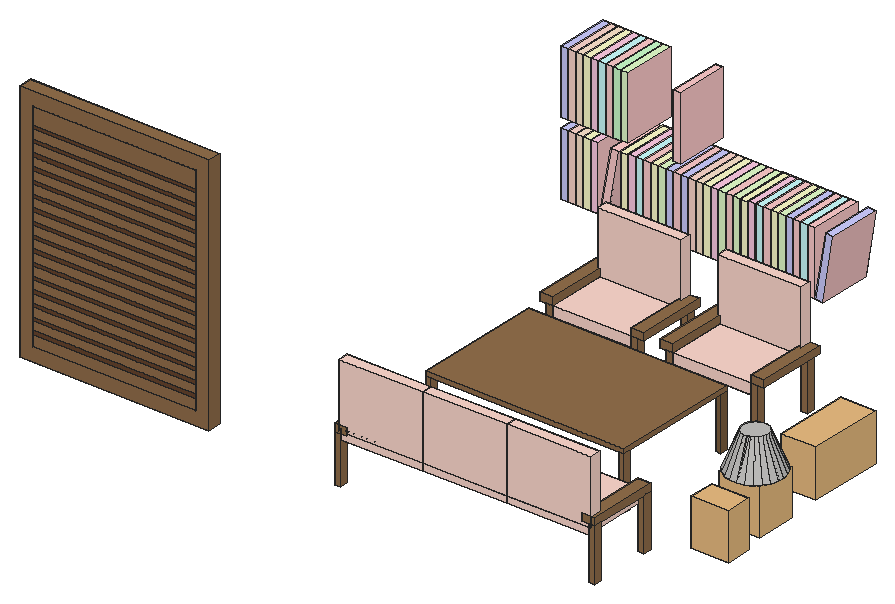
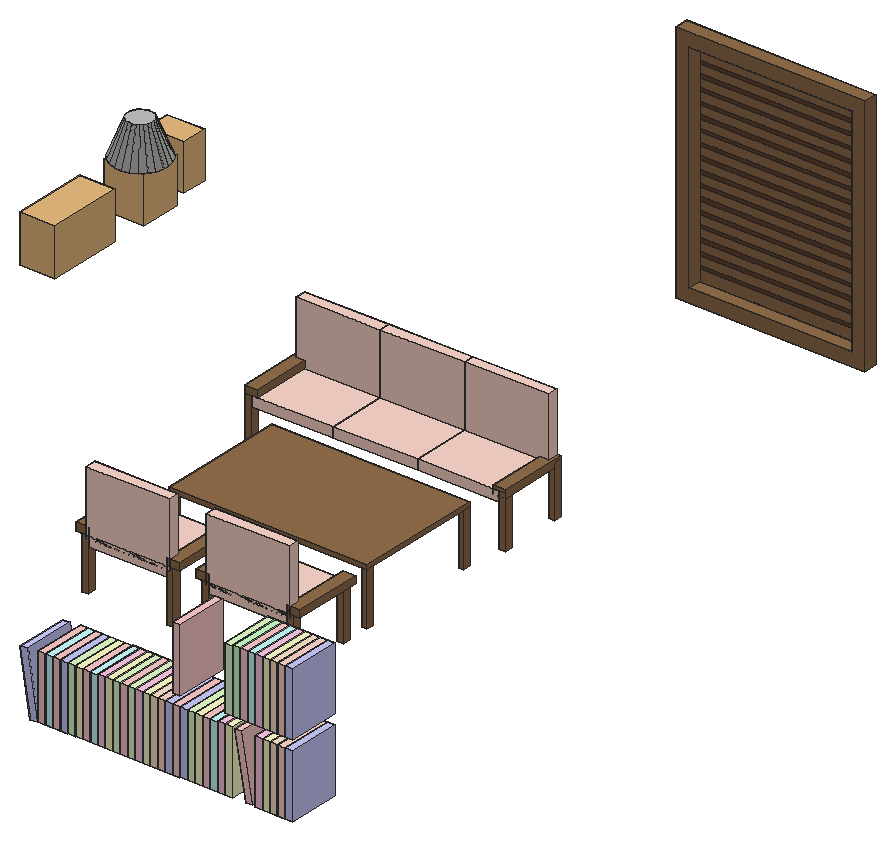
# SketchUp Ruby script. Lengths in inches.
U = 1.inch
M = Sketchup.active_model
def pt(a) = Geom::Point3d.new(a.map { |v| v * U })
def face(e, loops, mat)
  f = e.add_face(loops[0].map { |a| pt(a) })
  loops[1..].each { |l| e.add_face(l.map { |a| pt(a) }).erase! }
  f.material = f.back_material = mat if mat
  f
end
# faces: each face lists its corners as indices into pts; further lists are holes
def faces(e, pts, list, mat = nil) = list.each { |f| face(e, (f[0].is_a?(Array) ? f : [f]).map { |l| l.map { |i| pts[i] } }, mat) }
# xy, xz, yz: faces in a plane at the given z, y or x. An outline is a flat list of corners, or four numbers for a rectangle; further outlines are holes
def ring(l) = l.size == 4 ? [[l[0], l[1]], [l[2], l[1]], [l[2], l[3]], [l[0], l[3]]] : l.each_slice(2).to_a
def flat(e, list, mat, &to3) = list.each { |f| face(e, (f[0].is_a?(Array) ? f : [f]).map { |l| ring(l).map { |u, v| to3.(u, v) } }, mat) }
def xy(e, z, list, mat = nil) = flat(e, list, mat) { |x, y| [x, y, z] }
def xz(e, y, list, mat = nil) = flat(e, list, mat) { |x, z| [x, y, z] }
def yz(e, x, list, mat = nil) = flat(e, list, mat) { |y, z| [x, y, z] }
def lines(e, pts, list) = list.each { |a, b| e.add_line(pt(pts[a]), pt(pts[b])) }
# prism: a flat outline (further loops are holes) pulled along v
def prism(e, loops, v, mat = nil)
  f = face(e, loops, mat); d = Geom::Vector3d.new(v.map { |x| x * U })
  f.pushpull(f.normal.samedirection?(d) ? d.length : -d.length)
end
def box(e, o, s, mat = nil) = prism(e, [[o, [o[0] + s[0], o[1], o[2]], [o[0] + s[0], o[1] + s[1], o[2]], [o[0], o[1] + s[1], o[2]]]], [0, 0, s[2]], mat)
def at(x, y, z, deg = 0) = Geom::Transformation.translation(pt([x, y, z])) * Geom::Transformation.rotation(ORIGIN, Z_AXIS, deg.degrees)
def axes(o, x, y, z) = Geom::Transformation.new([*x, 0, *y, 0, *z, 0, *pt(o).to_a, 1])
def part(name) = M.definitions.add(name)
# library, detail: a bought-in or finely detailed component or shape, given as its bounding box
def library(name, o, s) = part(name).tap { |d| box(d.entities, o, s) }
def detail(e, o, s) = box(e.add_group.entities, o, s)
def put(e, d, t, mat = nil) = e.add_instance(d, t).tap { |i| i.material = mat if mat }
def group(e, t, mat = nil) = e.add_group.tap { |g| g.transformation = t; g.material = mat if mat }.entities
root = M.entities
M.materials.add("A01_Blush_Petal").color = [255, 204, 204]
M.materials.add("B01_Ivory_Dust").color = [255, 217, 206]
M.materials.add("Brick_Stack_Bond_2K2").color = [186, 186, 186]
M.materials.add("C01_Vanilla_Cream").color = [255, 230, 206]
M.materials.add("Carpet_01_1K").color = [196, 195, 193]
M.materials.add("Carpet_04_1K").color = [147, 87, 112]
M.materials.add("E01_Mint_Frost").color = [255, 255, 204]
M.materials.add("F01_Seafoam_Drift").color = [229, 255, 204]
M.materials.add("G01_Mint_Mist").color = [204, 255, 204]
M.materials.add("H01_Misty_Ice1").color = [204, 255, 255]
M.materials.add("I01_Sky_Frost").color = [204, 204, 255]
M.materials.add("L01_Cotton_Candy").color = [255, 204, 229]
M.materials.add("Plywood_01_1K").color = [125, 96, 64]
M.materials.add("Wood_Floor_01_1K").color = [146, 111, 76]
M.materials.add("Wood_Floor_01_1K1").color = [146, 111, 76]
M.materials.add("Wood_Veneer_15_1K").color = [103, 69, 45]
c1 = part("Group\#271")
xy(c1.entities,0,[[0,-3,42.6875,0]],"Wood_Floor_01_1K1")
xy(c1.entities,3,[[3,-3,39.6875,0]],"Wood_Floor_01_1K1")
xy(c1.entities,51.75,[[3,-3,39.6875,0]],"Wood_Floor_01_1K1")
xy(c1.entities,54.75,[[0,-3,42.6875,0]],"Wood_Floor_01_1K1")
xz(c1.entities,-3,[[[0,0,42.6875,54.75],[3,3,39.6875,51.75]],[3,3,39.6875,5.49],[3,6.39,39.6875,8.25],[3,9.15,39.6875,11.02],[3,11.92,39.6875,13.79],
  [3,14.6875,39.6875,16.55],[3,17.45,39.6875,19.32],[3,20.22,39.6875,22.09],[3,22.99,39.6875,24.85],[3,25.75,39.6875,27.62],
  [3,28.52,39.6875,30.39],[3,31.29,39.6875,33.15],[3,34.05,39.6875,35.92],[3,36.82,39.6875,38.6875],[3,39.59,39.6875,41.45],
  [3,42.35,39.6875,44.22],[3,45.12,39.6875,46.99],[3,47.89,39.6875,51.75]],"Wood_Floor_01_1K1")
xz(c1.entities,-3,[[3,5.49,39.6875,6.39],[3,8.25,39.6875,9.15],[3,11.02,39.6875,11.92],[3,13.79,39.6875,14.6875],[3,16.55,39.6875,17.45],
  [3,19.32,39.6875,20.22],[3,22.09,39.6875,22.99],[3,24.85,39.6875,25.75],[3,27.62,39.6875,28.52],[3,30.39,39.6875,31.29],
  [3,33.15,39.6875,34.05],[3,35.92,39.6875,36.82],[3,38.6875,39.6875,39.59],[3,41.45,39.6875,42.35],[3,44.22,39.6875,45.12],
  [3,46.99,39.6875,47.89]],"Wood_Veneer_15_1K")
xz(c1.entities,0,[[[0,0,42.6875,54.75],[3,3,39.6875,51.75]]],"Wood_Floor_01_1K1")
yz(c1.entities,0,[[-3,0,0,54.75]],"Wood_Floor_01_1K1")
yz(c1.entities,3,[[-3,3,0,51.75]],"Wood_Floor_01_1K1")
yz(c1.entities,39.6875,[[-3,3,0,51.75]],"Wood_Floor_01_1K1")
yz(c1.entities,42.6875,[[-3,0,0,54.75]],"Wood_Floor_01_1K1")
c2 = library("Group\#95",[0,0,0],[8.4375,5.8125,10.4375])
c3 = part("Group\#23")
box(c3.entities,[0,0,0],[1,1,7.4],"Wood_Floor_01_1K")
c4 = part("Group\#14")
box(c4.entities,[0,0,0],[1,1,7.4],"Wood_Floor_01_1K")
c5 = part("Group\#15")
box(c5.entities,[-0.4,-0.4,0],[12.8,1.4,9])
c6 = part("Group\#27")
box(c6.entities,[-2.93,0,0],[1.93,9,1.0625],"Wood_Floor_01_1K")
c7 = library("Group\#89",[0,0,0],[7.84,16.8125,10.71])
c8 = part("Group\#55")
box(c8.entities,[0,0,0],[1,1,7.4],"Wood_Floor_01_1K")
c9 = part("Group\#59")
box(c9.entities,[0,0,0],[1,1,7.4],"Wood_Floor_01_1K")
c10 = part("Group\#16")
box(c10.entities,[-2.93,0,0],[1.93,9,1.0625],"Wood_Floor_01_1K")
c11 = part("Group\#85")
xy(c11.entities,0,[[0,-12,1.73,0]])
xy(c11.entities,14.9,[[0,-12,1.73,0]])
xz(c11.entities,-12,[[0,0,1.73,14.9]],"I01_Sky_Frost")
xz(c11.entities,0,[[0,0,1.73,14.9]])
yz(c11.entities,0,[[-12,0,0,14.9]])
yz(c11.entities,1.73,[[-12,0,0,14.9]],"A01_Blush_Petal")
c12 = part("Group\#84")
xy(c12.entities,0,[[0,-12,1.73,0]])
xy(c12.entities,14.9,[[0,-12,1.73,0]])
xz(c12.entities,-12,[[0,0,1.73,14.9]],"A01_Blush_Petal")
xz(c12.entities,0,[[0,0,1.73,14.9]])
yz(c12.entities,0,[[-12,0,0,14.9]])
yz(c12.entities,1.73,[[-12,0,0,14.9]],"A01_Blush_Petal")
c13 = part("Group\#22")
xy(c13.entities,0,[[0,-12,1.73,0]])
xy(c13.entities,14.9,[[0,-12,1.73,0]],"C01_Vanilla_Cream")
xz(c13.entities,-12,[[0,0,1.73,14.9]],"C01_Vanilla_Cream")
xz(c13.entities,0,[[0,0,1.73,14.9]])
yz(c13.entities,0,[[-12,0,0,14.9]])
yz(c13.entities,1.73,[[-12,0,0,14.9]],"C01_Vanilla_Cream")
c14 = part("Group\#60")
xy(c14.entities,0,[[0,-12,1.73,0]])
xy(c14.entities,14.9,[[0,-12,1.73,0]])
xz(c14.entities,-12,[[0,0,1.73,14.9]],"B01_Ivory_Dust")
xz(c14.entities,0,[[0,0,1.73,14.9]])
yz(c14.entities,0,[[-12,0,0,14.9]])
yz(c14.entities,1.73,[[-12,0,0,14.9]],"A01_Blush_Petal")
c15 = part("Group\#83")
xy(c15.entities,0,[[0,-12,1.73,0]])
xy(c15.entities,14.9,[[0,-12,1.73,0]])
xz(c15.entities,-12,[[0,0,1.73,14.9]],"E01_Mint_Frost")
xz(c15.entities,0,[[0,0,1.73,14.9]])
yz(c15.entities,0,[[-12,0,0,14.9]])
yz(c15.entities,1.73,[[-12,0,0,14.9]],"A01_Blush_Petal")
c16 = part("Group\#66")
xy(c16.entities,0,[[0,-12,1.73,0]])
xy(c16.entities,14.9,[[0,-12,1.73,0]],"L01_Cotton_Candy")
xz(c16.entities,-12,[[0,0,1.73,14.9]],"L01_Cotton_Candy")
xz(c16.entities,0,[[0,0,1.73,14.9]])
yz(c16.entities,0,[[-12,0,0,14.9]])
yz(c16.entities,1.73,[[-12,0,0,14.9]],"A01_Blush_Petal")
c17 = part("Group\#71")
xy(c17.entities,0,[[0,-12,1.73,0]])
xy(c17.entities,14.9,[[0,-12,1.73,0]])
xz(c17.entities,-12,[[0,0,1.73,14.9]],"F01_Seafoam_Drift")
xz(c17.entities,0,[[0,0,1.73,14.9]])
yz(c17.entities,0,[[-12,0,0,14.9]])
yz(c17.entities,1.73,[[-12,0,0,14.9]],"A01_Blush_Petal")
c18 = part("Group\#69")
xy(c18.entities,0,[[0,-12,1.73,0]])
xy(c18.entities,14.9,[[0,-12,1.73,0]])
xz(c18.entities,-12,[[0,0,1.73,14.9]],"H01_Misty_Ice1")
xz(c18.entities,0,[[0,0,1.73,14.9]])
yz(c18.entities,0,[[-12,0,0,14.9]])
yz(c18.entities,1.73,[[-12,0,0,14.9]],"A01_Blush_Petal")
c19 = part("Group\#62")
xy(c19.entities,0,[[0,-12,1.73,0]])
xy(c19.entities,14.9,[[0,-12,1.73,0]])
xz(c19.entities,-12,[[0,0,1.73,14.9]],"F01_Seafoam_Drift")
xz(c19.entities,0,[[0,0,1.73,14.9]])
yz(c19.entities,0,[[-12,0,0,14.9]])
yz(c19.entities,1.73,[[-12,0,0,14.9]],"A01_Blush_Petal")
c20 = part("Group\#63")
xy(c20.entities,0,[[0,-12,1.73,0]])
xy(c20.entities,14.9,[[0,-12,1.73,0]])
xz(c20.entities,-12,[[0,0,1.73,14.9]],"G01_Mint_Mist")
xz(c20.entities,0,[[0,0,1.73,14.9]])
yz(c20.entities,0,[[-12,0,0,14.9]])
yz(c20.entities,1.73,[[-12,0,0,14.9]],"A01_Blush_Petal")
put(root,c1,at(1653.9375,215.6875,47.25))
put(root,c2,at(1788.49,233.81,46.58))
g1 = group(root,at(1786.57,244.02,46.58),"Wood_Floor_01_1K1")
xy(g1,10.4375,[[[5.244,-1.427,6.781,-1.055,8.17,-0.297,9.316,0.794,10.14,2.144,10.586,3.662,10.624,5.244,10.252,6.781,9.495,8.17,8.403,9.316,7.053,10.14,5.535,10.586,3.954,10.624,2.416,10.252,1.027,9.495,-0.118,8.403,-0.942,7.053,-1.389,5.535,-1.427,3.954,-1.055,2.416,-0.297,1.027,0.794,-0.118,2.144,-0.942,3.662,-1.389],[5.241,-1.404,3.666,-1.366,2.154,-0.921,0.808,-0.1,-0.279,1.041,-1.033,2.424,-1.404,3.956,-1.366,5.532,-0.921,7.044,-0.1,8.389,1.041,9.476,2.424,10.231,3.956,10.602,5.532,10.563,7.044,10.119,8.389,9.298,9.476,8.157,10.231,6.773,10.602,5.241,10.563,3.666,10.119,2.154,9.298,0.808,8.157,-0.279,6.773,-1.033,5.244,-1.404]]],"Carpet_01_1K")
xy(g1,18.4375,[[5.321,1.769,5.324,1.881,5.62,1.953,6.27,2.308,6.806,2.818,7.192,3.45,7.401,4.16,7.419,4.901,7.244,5.62,6.89,6.27,6.379,6.806,5.747,7.192,5.037,7.401,4.297,7.419,3.577,7.244,2.927,6.89,2.391,6.379,2.006,5.747,1.797,5.037,1.779,4.297,1.953,3.577,2.308,2.927,2.818,2.391,3.45,2.006,4.16,1.797,4.901,1.779]],"Carpet_01_1K")
p = [[3.666,-1.366,10.4375],[4.16,1.797,18.4375],[3.45,2.006,18.4375],[2.154,-0.921,10.4375],[5.244,-1.404,10.4375],[5.321,1.769,18.4375],
  [4.901,1.779,18.4375],[5.241,-1.404,10.4375],[6.773,-1.033,10.4375],[5.62,1.953,18.4375],[5.324,1.881,18.4375],[8.157,-0.279,10.4375],
  [6.27,2.308,18.4375],[2.818,2.391,18.4375],[0.808,-0.1,10.4375],[9.298,0.808,10.4375],[6.806,2.818,18.4375],[2.308,2.927,18.4375],
  [-0.279,1.041,10.4375],[10.119,2.154,10.4375],[7.192,3.45,18.4375],[1.953,3.577,18.4375],[-1.033,2.424,10.4375],[10.563,3.666,10.4375],
  [7.401,4.16,18.4375],[1.779,4.297,18.4375],[-1.404,3.956,10.4375],[10.602,5.241,10.4375],[7.419,4.901,18.4375],[1.797,5.037,18.4375],
  [-1.366,5.532,10.4375],[10.231,6.773,10.4375],[7.244,5.62,18.4375],[2.006,5.747,18.4375],[-0.921,7.044,10.4375],[9.476,8.157,10.4375],
  [6.89,6.27,18.4375],[2.391,6.379,18.4375],[-0.1,8.389,10.4375],[8.389,9.298,10.4375],[6.379,6.806,18.4375],[2.927,6.89,18.4375],
  [1.041,9.476,10.4375],[7.044,10.119,10.4375],[5.747,7.192,18.4375],[3.577,7.244,18.4375],[2.424,10.231,10.4375],[4.297,7.419,18.4375],
  [3.956,10.602,10.4375],[5.532,10.563,10.4375],[5.037,7.401,18.4375],[5.39,4.58,10.4375],[5.387,4.475,10.4375],[4.599,4.599,10.4375],
  [5.242,4.583,10.4375]]
faces(g1,p,[[0,1,2,3],[4,5,6,1,0,7],[8,9,10,6,7,4],[11,12,9,8],[3,2,13,14],[15,16,12,11],[14,13,17,18],[19,20,16,15],
  [18,17,21,22],[23,24,20,19],[22,21,25,26],[27,28,24,23],[26,25,29,30],[31,32,28,27],[30,29,33,34],[35,36,32,31],
  [34,33,37,38],[39,40,36,35],[38,37,41,42],[43,44,40,39],[42,41,45,46],[46,45,47,48],[49,50,44,43],[48,47,50,49]],"Carpet_01_1K")
lines(g1,p,[[51,52],[53,54],[54,51]])
detail(g1,[0,0,0],[9.2,9.2,10.4375])
g2 = group(root,at(1715.03,266.69,19),"Brick_Stack_Bond_2K2")
g3 = group(g2,at(-1.47,-0.01,9.59),"B01_Ivory_Dust")
xy(g3,0,[[-17.53,-16.01,-17.68,-0.17,0.59,0.01,0.74,-15.83]],"B01_Ivory_Dust")
xy(g3,2.24,[[-17.53,-16.01,0.74,-15.83,0.59,0.01,-17.68,-0.17]],"B01_Ivory_Dust")
p = [[-17.68,-0.17,0],[-17.53,-16.01,0],[-17.53,-16.01,2.24],[-17.68,-0.17,2.24],[0.74,-15.83,0],[0.74,-15.83,2.24],
  [0.59,0.01,0],[0.59,0.01,2.24]]
faces(g3,p,[[0,1,2,3],[1,4,5,2],[6,0,3,7]],"B01_Ivory_Dust")
faces(g3,p,[[6,7,5,4]],"Carpet_04_1K")
put(g2,c3,axes([-19.02,-14.26,0],[-1.47313,-0.01417,0],[0.01693,-1.75992,0],[0,0,1.599]))
put(g2,c4,axes([-19.15,-0.18,0],[-1.47313,-0.01417,0],[0.01693,-1.75992,0],[0,0,1.599]))
put(g2,c5,axes([-1.34,-14.09,11.19],[-1.47313,-0.01417,0],[0.01693,-1.75992,0],[0,0,1.599]),"B01_Ivory_Dust")
put(g2,c6,axes([-22.1,-0.21,10.73],[-1.47313,-0.01417,0],[0.01693,-1.75992,0],[0,0,1.599]))
g4 = group(g2,at(17.38,0.17,9.59),"B01_Ivory_Dust")
xy(g4,0,[[-18.11,-16.01,-18.27,-0.18,0.59,0.01,0.74,-15.83]],"B01_Ivory_Dust")
xy(g4,2.24,[[-18.11,-16.01,0.74,-15.83,0.59,0.01,-18.27,-0.18]],"B01_Ivory_Dust")
p = [[-18.27,-0.18,0],[-18.11,-16.01,0],[-18.11,-16.01,2.24],[-18.27,-0.18,2.24],[0.74,-15.83,0],[0.74,-15.83,2.24],
  [0.59,0.01,0],[0.59,0.01,2.24]]
faces(g4,p,[[0,1,2,3],[6,7,5,4]],"Carpet_04_1K")
faces(g4,p,[[1,4,5,2],[6,0,3,7]],"B01_Ivory_Dust")
put(g2,c5,axes([17.52,-13.91,11.19],[-1.47313,-0.01417,0],[0.01693,-1.75992,0],[0,0,1.599]),"B01_Ivory_Dust")
g5 = group(g2,at(36.24,0.35,9.59),"Carpet_01_1K")
xy(g5,0,[[-18.11,-16.01,-18.27,-0.18,0,0,0.15,-15.84]],"B01_Ivory_Dust")
xy(g5,2.24,[[-18.11,-16.01,0.15,-15.84,0,0,-18.27,-0.18]],"B01_Ivory_Dust")
p = [[-18.27,-0.18,0],[-18.11,-16.01,0],[-18.11,-16.01,2.24],[-18.27,-0.18,2.24],[0.15,-15.84,0],[0.15,-15.84,2.24],
  [0,0,0],[0,0,2.24]]
faces(g5,p,[[0,1,2,3]],"Carpet_04_1K")
faces(g5,p,[[1,4,5,2],[6,7,5,4],[6,0,3,7]],"B01_Ivory_Dust")
put(g2,c5,axes([36.375,-13.73,11.19],[-1.47313,-0.01417,0],[0.01693,-1.75992,0],[0,0,1.599]),"B01_Ivory_Dust")
put(g2,c6,axes([33.39,0.32,11.83],[-1.47313,-0.01417,0],[0.01693,-1.75992,0],[0,0,1.599]))
put(g2,c3,axes([37.85,-13.72,0],[-1.47313,-0.01417,0],[0.01693,-1.75992,0],[0,0,1.599]))
put(g2,c4,axes([37.71,0.36,0],[-1.47313,-0.01417,0],[0.01693,-1.75992,0],[0,0,1.599]))
put(root,c7,at(1787.125,260.92,46.58))
g6 = group(root,at(1696.03,274.53,19),"Wood_Floor_01_1K")
g7 = group(g6,at(0,27.38,0))
xy(g7,0,[[0,0,1.24,1.61]],"Plywood_01_1K")
xy(g7,12,[[0,0,1.24,1.61]],"Plywood_01_1K")
xz(g7,0,[[0,0,1.24,12]],"Wood_Floor_01_1K")
xz(g7,1.61,[[0,0,1.24,12]],"Wood_Floor_01_1K")
yz(g7,0,[[0,0,1.61,12]],"Wood_Floor_01_1K")
yz(g7,1.24,[[0,0,1.61,12]],"Wood_Floor_01_1K")
g8 = group(g6,at(43.49,27.38,0))
box(g8,[0,0,0],[1.24,1.61,12],"Plywood_01_1K")
g9 = group(g6,at(43.49,0,0))
xy(g9,0,[[0,0,1.24,1.61]],"Plywood_01_1K")
xy(g9,12,[[0,0,1.24,1.61]],"Plywood_01_1K")
xz(g9,0,[[0,0,1.24,12]],"Wood_Floor_01_1K")
xz(g9,1.61,[[0,0,1.24,12]],"Wood_Floor_01_1K")
yz(g9,0,[[0,0,1.61,12]],"Wood_Floor_01_1K")
yz(g9,1.24,[[0,0,1.61,12]],"Wood_Floor_01_1K")
g10 = group(g6,at(0,0,0),"Wood_Floor_01_1K")
xy(g10,0,[[0,0,1.24,1.61]],"Plywood_01_1K")
xy(g10,12,[[0,0,1.24,1.61]],"Plywood_01_1K")
xz(g10,0,[[0,0,1.24,12]],"Wood_Floor_01_1K")
xz(g10,1.61,[[0,0,1.24,12]],"Wood_Floor_01_1K")
yz(g10,0,[[0,0,1.61,12]],"Wood_Floor_01_1K")
yz(g10,1.24,[[0,0,1.61,12]],"Wood_Floor_01_1K")
g11 = group(g6,at(0,0,12),"Plywood_01_1K")
xy(g11,1,[[0,0,44.73,28.99]],"Wood_Floor_01_1K")
xz(g11,0,[[0,0,44.73,1]],"Wood_Floor_01_1K")
xz(g11,28.99,[[0,0,44.73,1]],"Wood_Floor_01_1K")
yz(g11,0,[[0,0,28.99,1]],"Wood_Floor_01_1K")
yz(g11,44.73,[[0,0,28.99,1]],"Wood_Floor_01_1K")
g12 = group(root,at(1696.03,308.48,19),"Brick_Stack_Bond_2K2")
g13 = group(g12,at(1.47,0,9.59),"B01_Ivory_Dust")
box(g13,[0,0,0],[17.68,15.84,2.24],"B01_Ivory_Dust")
put(g12,c8,axes([0,0,0],[1.4732,0,0],[0,1.76,0],[0,0,1.599]))
put(g12,c9,axes([0,14.08,0],[1.4732,0,0],[0,1.76,0],[0,0,1.599]))
put(g12,c3,axes([19.15,14.08,0],[1.4732,0,0],[0,1.76,0],[0,0,1.599]))
put(g12,c10,axes([2.95,0,11.83],[1.4732,0,0],[0,1.76,0],[0,0,1.599]))
put(g12,c4,axes([19.15,0,0],[1.4732,0,0],[0,1.76,0],[0,0,1.599]))
put(g12,c5,axes([1.47,14.08,11.19],[1.4732,0,0],[0,1.76,0],[0,0,1.599]),"B01_Ivory_Dust")
put(g12,c6,axes([23.47,0,11.83],[1.4732,0,0],[0,1.76,0],[0,0,1.599]))
g14 = group(root,at(1723.15,308.48,19),"Brick_Stack_Bond_2K2")
g15 = group(g14,at(1.47,0,9.59),"B01_Ivory_Dust")
box(g15,[0,0,0],[17.68,15.84,2.24],"B01_Ivory_Dust")
put(g14,c8,axes([0,0,0],[1.4732,0,0],[0,1.76,0],[0,0,1.599]))
put(g14,c9,axes([0,14.08,0],[1.4732,0,0],[0,1.76,0],[0,0,1.599]))
put(g14,c3,axes([19.15,14.08,0],[1.4732,0,0],[0,1.76,0],[0,0,1.599]))
put(g14,c10,axes([2.95,0,11.83],[1.4732,0,0],[0,1.76,0],[0,0,1.599]))
put(g14,c4,axes([19.15,0,0],[1.4732,0,0],[0,1.76,0],[0,0,1.599]))
put(g14,c5,axes([1.47,14.08,11.19],[1.4732,0,0],[0,1.76,0],[0,0,1.599]),"B01_Ivory_Dust")
put(g14,c6,axes([23.47,0,11.83],[1.4732,0,0],[0,1.76,0],[0,0,1.599]))
put(root,c11,axes([1719.76,366.75,19.74],[0.98625,0,-0.16523],[0,1,0],[0.15862,0,0.9468]),"I01_Sky_Frost")
put(root,c12,axes([1671.17,366.75,20.01],[0.98389,0,-0.1788],[0,1,0],[0.17165,0,0.94453]),"A01_Blush_Petal")
put(root,c13,axes([1665.69,366.75,19.74],[1,0,0],[0,1,0],[0,0,0.96]),"C01_Vanilla_Cream")
put(root,c11,axes([1662.31,366.75,19.74],[1,0,0],[0,1,0],[0,0,0.96]),"I01_Sky_Frost")
put(root,c14,axes([1664,366.75,19.74],[1,0,0],[0,1,0],[0,0,0.96]),"B01_Ivory_Dust")
put(root,c15,axes([1675.81,366.75,19.74],[1,0,0],[0,1,0],[0,0,0.96]),"E01_Mint_Frost")
put(root,c12,axes([1687.63,366.75,19.74],[1,0,0],[0,1,0],[0,0,0.96]),"A01_Blush_Petal")
put(root,c15,axes([1667.38,366.75,19.74],[1,0,0],[0,1,0],[0,0,0.96]),"E01_Mint_Frost")
put(root,c16,axes([1669.06,366.75,19.74],[1,0,0],[0,1,0],[0,0,0.96]),"L01_Cotton_Candy")
put(root,c12,axes([1680.88,366.75,19.74],[1,0,0],[0,1,0],[0,0,0.96]),"A01_Blush_Petal")
put(root,c17,axes([1684.25,366.75,19.74],[1,0,0],[0,1,0],[0,0,0.96]),"F01_Seafoam_Drift")
put(root,c16,axes([1677.5,366.75,19.74],[1,0,0],[0,1,0],[0,0,0.96]),"L01_Cotton_Candy")
put(root,c18,axes([1679.19,366.75,19.74],[1,0,0],[0,1,0],[0,0,0.96]),"H01_Misty_Ice1")
put(root,c11,axes([1685.98,366.75,19.74],[1,0,0],[0,1,0],[0,0,0.96]),"I01_Sky_Frost")
put(root,c14,axes([1691.04,366.75,19.74],[1,0,0],[0,1,0],[0,0,0.96]),"B01_Ivory_Dust")
put(root,c16,axes([1696.1,366.75,19.74],[1,0,0],[0,1,0],[0,0,0.96]),"L01_Cotton_Candy")
put(root,c12,axes([1699.48,366.75,19.74],[1,0,0],[0,1,0],[0,0,0.96]),"A01_Blush_Petal")
put(root,c16,axes([1704.54,366.75,19.74],[1,0,0],[0,1,0],[0,0,0.96]),"L01_Cotton_Candy")
put(root,c12,axes([1714.66,366.75,19.74],[1,0,0],[0,1,0],[0,0,0.96]),"A01_Blush_Petal")
put(root,c12,axes([1707.91,366.75,19.74],[1,0,0],[0,1,0],[0,0,0.96]),"A01_Blush_Petal")
put(root,c17,axes([1711.29,366.75,19.74],[1,0,0],[0,1,0],[0,0,0.96]),"F01_Seafoam_Drift")
put(root,c18,axes([1706.23,366.75,19.74],[1,0,0],[0,1,0],[0,0,0.96]),"H01_Misty_Ice1")
put(root,c15,axes([1694.41,366.75,19.74],[1,0,0],[0,1,0],[0,0,0.96]),"E01_Mint_Frost")
put(root,c11,axes([1689.35,366.75,19.74],[1,0,0],[0,1,0],[0,0,0.96]),"I01_Sky_Frost")
put(root,c15,axes([1702.85,366.75,19.74],[1,0,0],[0,1,0],[0,0,0.96]),"E01_Mint_Frost")
put(root,c11,axes([1713.01,366.75,19.74],[1,0,0],[0,1,0],[0,0,0.96]),"I01_Sky_Frost")
put(root,c13,axes([1692.73,366.75,19.74],[1,0,0],[0,1,0],[0,0,0.96]),"C01_Vanilla_Cream")
put(root,c19,axes([1697.79,366.75,19.74],[1,0,0],[0,1,0],[0,0,0.96]),"F01_Seafoam_Drift")
put(root,c19,axes([1701.2,366.75,19.74],[1,0,0],[0,1,0],[0,0,0.96]),"F01_Seafoam_Drift")
put(root,c15,axes([1682.6,366.75,19.74],[1,0,0],[0,1,0],[0,0,0.96]),"E01_Mint_Frost")
put(root,c15,axes([1709.64,366.75,19.74],[1,0,0],[0,1,0],[0,0,0.96]),"E01_Mint_Frost")
put(root,c12,axes([1718.04,366.75,19.74],[1,0,0],[0,1,0],[0,0,0.96]),"A01_Blush_Petal")
put(root,c18,axes([1716.35,366.75,19.74],[1,0,0],[0,1,0],[0,0,0.96]),"H01_Misty_Ice1")
put(root,c11,axes([1662.31,366.75,36.28],[1,0,0],[0,1,0],[0,0,0.96]),"I01_Sky_Frost")
put(root,c14,axes([1664,366.75,36.28],[1,0,0],[0,1,0],[0,0,0.96]),"B01_Ivory_Dust")
put(root,c13,axes([1665.69,366.75,36.28],[1,0,0],[0,1,0],[0,0,0.96]),"C01_Vanilla_Cream")
put(root,c15,axes([1667.38,366.75,36.28],[1,0,0],[0,1,0],[0,0,0.96]),"E01_Mint_Frost")
put(root,c16,axes([1669.06,366.75,36.28],[1,0,0],[0,1,0],[0,0,0.96]),"L01_Cotton_Candy")
put(root,c18,axes([1670.75,366.75,36.28],[1,0,0],[0,1,0],[0,0,0.96]),"H01_Misty_Ice1")
put(root,c12,axes([1672.44,366.75,36.28],[1,0,0],[0,1,0],[0,0,0.96]),"A01_Blush_Petal")
put(root,c20,axes([1674.13,366.75,36.28],[1,0,0],[0,1,0],[0,0,0.96]),"G01_Mint_Mist")
put(root,c19,axes([1675.81,366.75,36.28],[1,0,0],[0,1,0],[0,0,0.96]),"F01_Seafoam_Drift")
put(root,c12,axes([1687.63,366.75,36.28],[1,0,0],[0,1,0],[0,0,0.96]),"A01_Blush_Petal")
